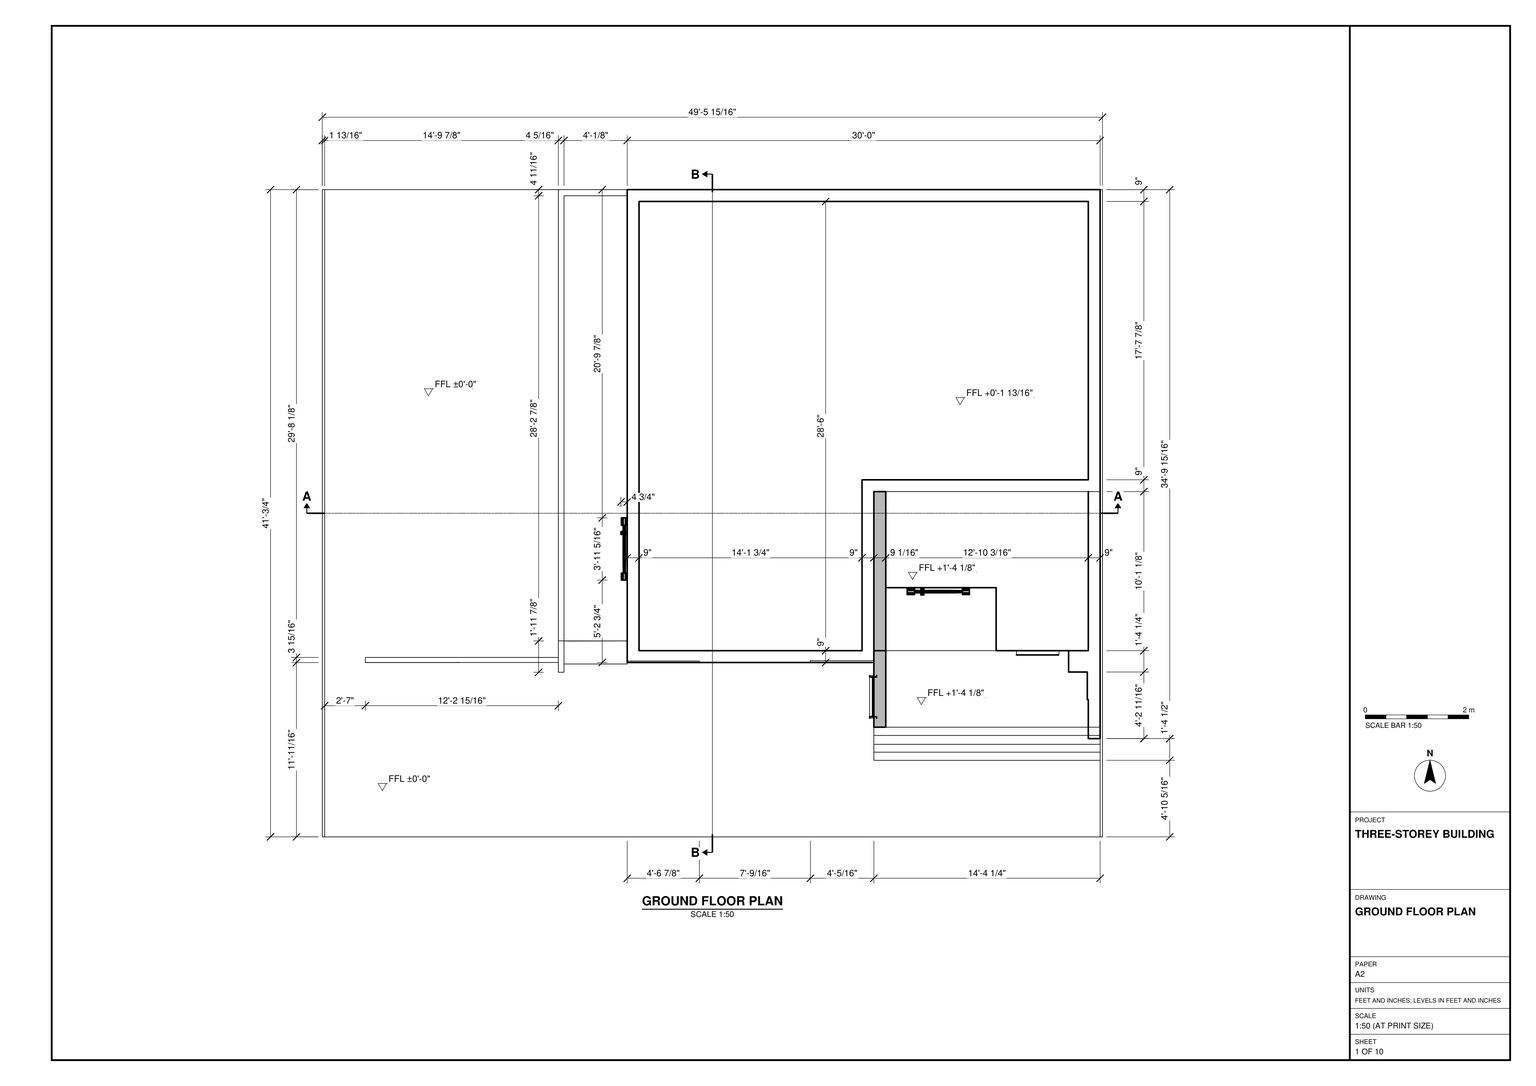
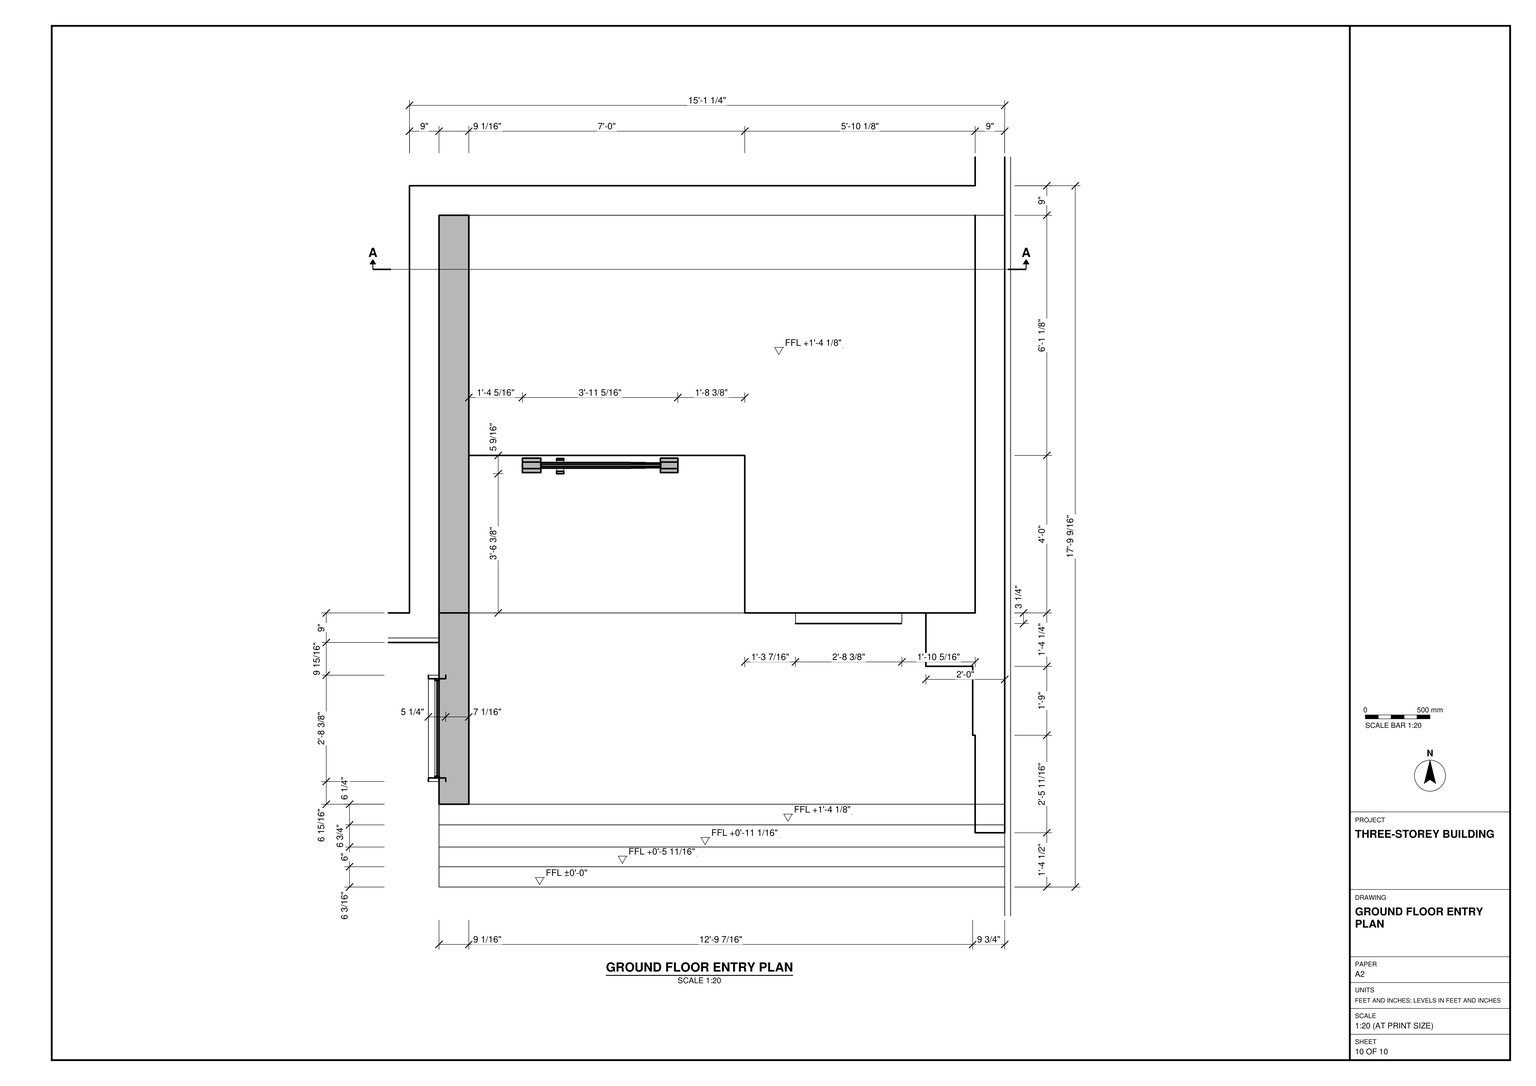
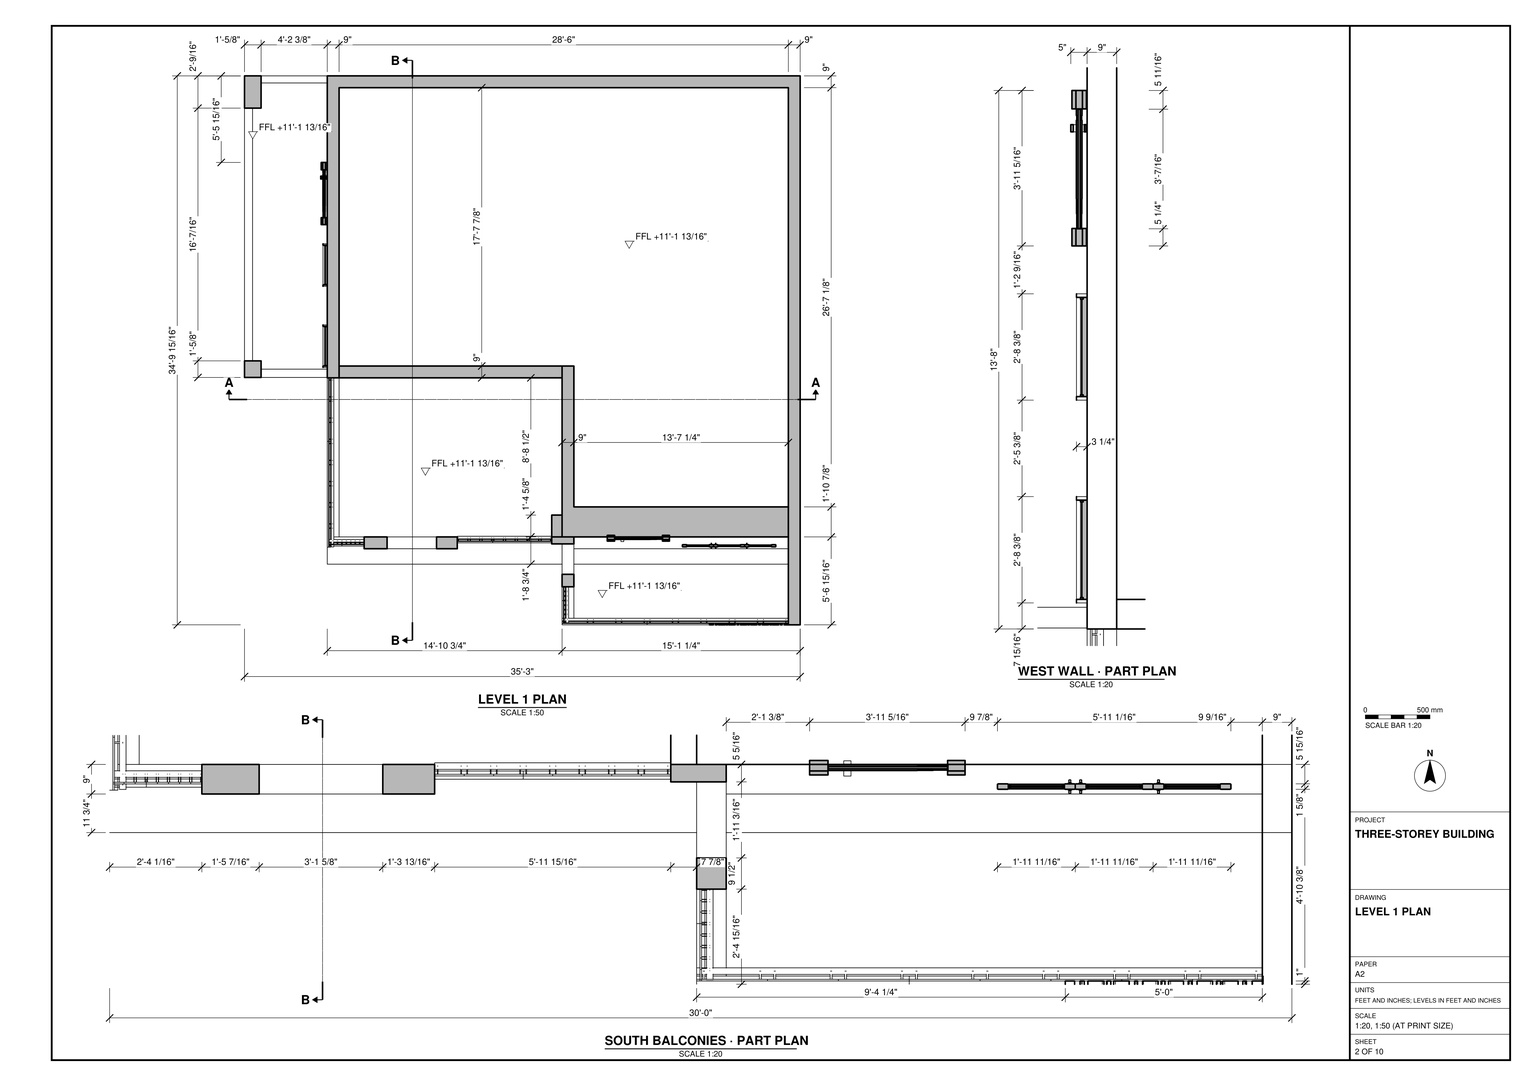
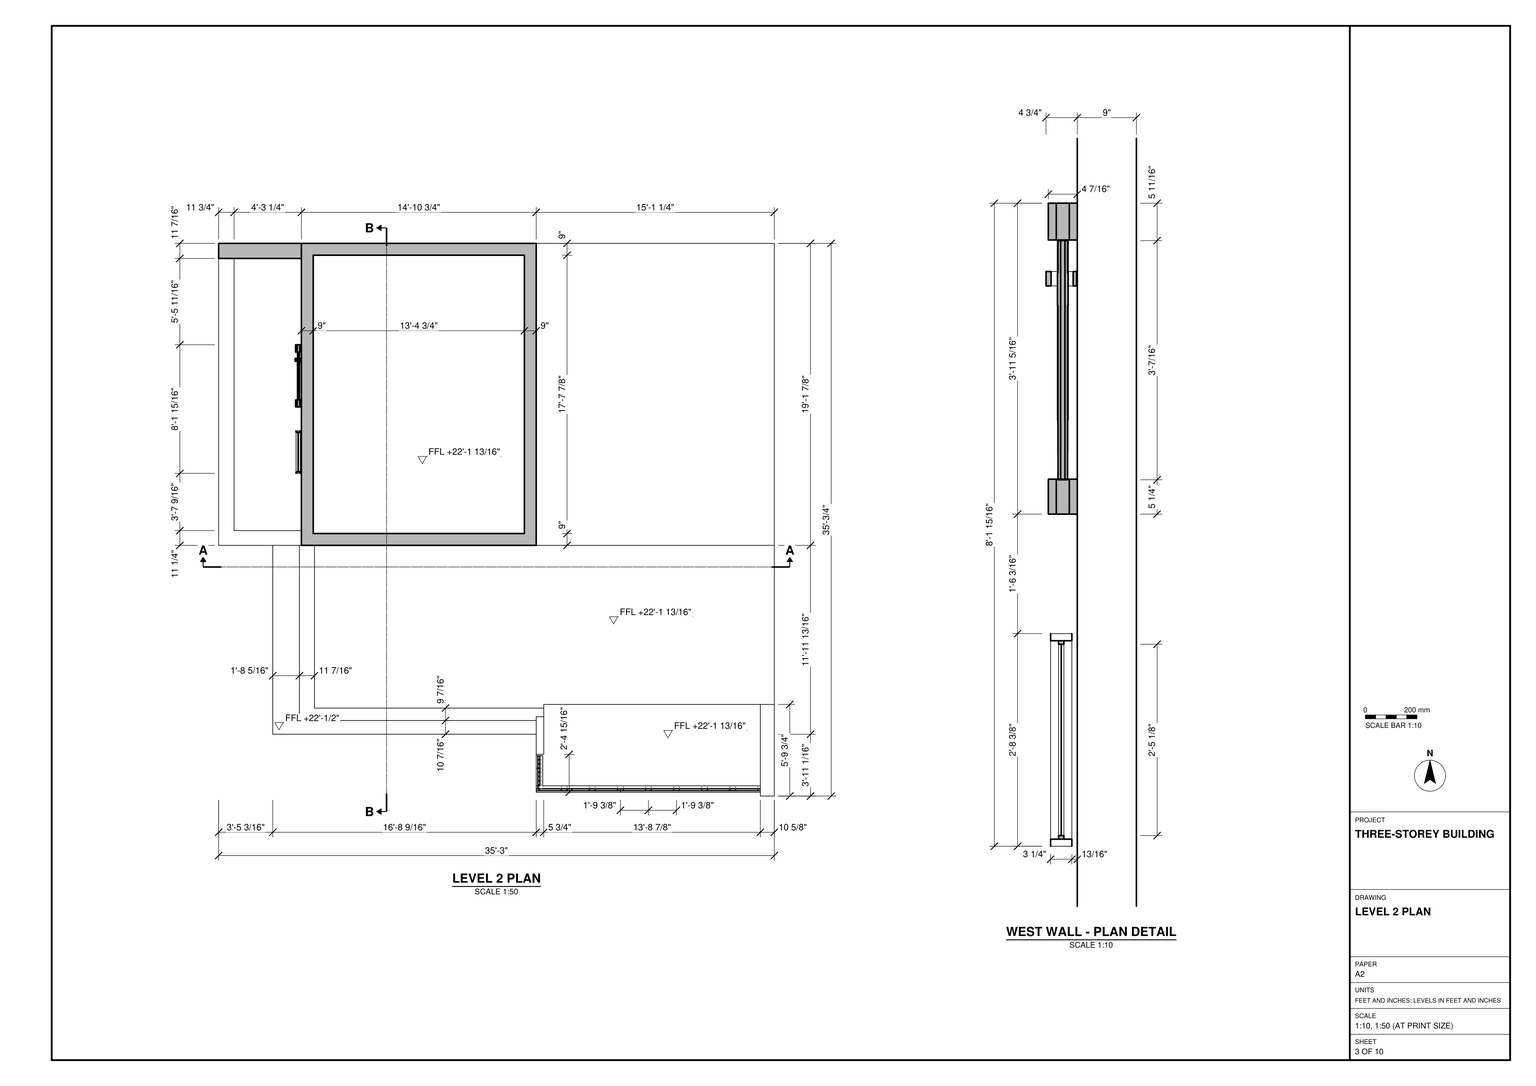
Build the three-storey building and its surrounding ground in SketchUp using task_files/diagram_01.pdf. Work in feet and inches. The overall model, including the ground shown in plan, measures 49'-5 15/16" along x, 41'-3/4" along y and 34'-0" along z. Use ±0'-0" as the ground datum and set the upper floor levels at +11'-1 13/16" and +22'-1 13/16".

Place the building on the east side of the ground plan, leaving the open area to the west. Use the enlarged entry plan to shape the south approach, steps and raised landing. Model the slabs and walls with their offsets, returns and thicknesses as drawn. On Level 1, follow the L-shaped enclosed area and the staggered outlines of the south balconies. Use the part plans to position the balcony guards, doors and window units. Follow the sheets for the uppermost storey, roof, stairs and any built-in joinery or main furniture shown. Suitable library components may be used for decor and loose items.

Keep shell elements such as walls, slabs and roof separate as groups or components. Do the same for each furniture or joinery piece, and use components for repeated parts. Save one SketchUp model as output_files/three_storey_building_with_south_balconies.skp.

# SketchUp Ruby script. Lengths in inches.
U = 1.inch
M = Sketchup.active_model
def pt(a) = Geom::Point3d.new(a.map { |v| v * U })
def face(e, loops, mat)
  f = e.add_face(loops[0].map { |a| pt(a) })
  loops[1..].each { |l| e.add_face(l.map { |a| pt(a) }).erase! }
  f.material = f.back_material = mat if mat
  f
end
# faces: each face lists its corners as indices into pts; further lists are holes
def faces(e, pts, list, mat = nil) = list.each { |f| face(e, (f[0].is_a?(Array) ? f : [f]).map { |l| l.map { |i| pts[i] } }, mat) }
# xy, xz, yz: faces in a plane at the given z, y or x. An outline is a flat list of corners, or four numbers for a rectangle; further outlines are holes
def ring(l) = l.size == 4 ? [[l[0], l[1]], [l[2], l[1]], [l[2], l[3]], [l[0], l[3]]] : l.each_slice(2).to_a
def flat(e, list, mat, &to3) = list.each { |f| face(e, (f[0].is_a?(Array) ? f : [f]).map { |l| ring(l).map { |u, v| to3.(u, v) } }, mat) }
def xy(e, z, list, mat = nil) = flat(e, list, mat) { |x, y| [x, y, z] }
def xz(e, y, list, mat = nil) = flat(e, list, mat) { |x, z| [x, y, z] }
def yz(e, x, list, mat = nil) = flat(e, list, mat) { |y, z| [x, y, z] }
def lines(e, pts, list) = list.each { |a, b| e.add_line(pt(pts[a]), pt(pts[b])) }
# prism: a flat outline (further loops are holes) pulled along v
def prism(e, loops, v, mat = nil)
  f = face(e, loops, mat); d = Geom::Vector3d.new(v.map { |x| x * U })
  f.pushpull(f.normal.samedirection?(d) ? d.length : -d.length)
end
def box(e, o, s, mat = nil) = prism(e, [[o, [o[0] + s[0], o[1], o[2]], [o[0] + s[0], o[1] + s[1], o[2]], [o[0], o[1] + s[1], o[2]]]], [0, 0, s[2]], mat)
def at(x, y, z, deg = 0) = Geom::Transformation.translation(pt([x, y, z])) * Geom::Transformation.rotation(ORIGIN, Z_AXIS, deg.degrees)
def axes(o, x, y, z) = Geom::Transformation.new([*x, 0, *y, 0, *z, 0, *pt(o).to_a, 1])
def part(name) = M.definitions.add(name)
# library, detail: a bought-in or finely detailed component or shape, given as its bounding box
def library(name, o, s) = part(name).tap { |d| box(d.entities, o, s) }
def detail(e, o, s) = box(e.add_group.entities, o, s)
def put(e, d, t, mat = nil) = e.add_instance(d, t).tap { |i| i.material = mat if mat }
def group(e, t, mat = nil) = e.add_group.tap { |g| g.transformation = t; g.material = mat if mat }.entities
root = M.entities
M.materials.add("[Color M00]1").color = [255, 255, 255]
M.materials.add("[Color M04]").color = [142, 142, 142]
M.materials.add("[Color M05]1").color = [114, 114, 114]
M.materials.add("[Color M06]").color = [86, 86, 86]
M.materials.add("[Color M08]1").color = [30, 30, 30]
M.materials.add("[Color M09]1").color = [0, 0, 0]
M.materials.add("[Wood Cherry Original]").color = [152, 86, 42]
M.materials.add("[Wood Floor Light]").color = [204, 176, 127]
M.materials.add("[Wood Veneer 01]").color = [120, 70, 37]
c1 = library("Three panel window",[0,0,0],[5.02,84.63,60])
c2 = library("PORTA PIVOTANTE D luxury",[0,-0.8125,0],[63.375,11.25,89])
c3 = library("Single panel window",[84,-6,0],[60,6,73.01])
c4 = library("Untitled",[0,0,0],[571,5,42])
c5 = library("jali pattern 5",[0,0,0],[60,1,120])
c6 = part("Group\#2")
xy(c6.entities,0,[[-232.125,-492.75,360,0]])
xy(c6.entities,10.1875,[[-232.125,-492.75,360,0]])
xz(c6.entities,-492.75,[[-232.125,0,360,10.1875]],"[Color M05]1")
xz(c6.entities,0,[[-232.125,0,360,10.1875]])
yz(c6.entities,-232.125,[[-492.75,0,0,10.1875]])
yz(c6.entities,360,[[-492.75,0,0,10.1875]])
c7 = part("Group\#7")
box(c7.entities,[0,0,0],[1.0625,3.0625,13.875])
xy(root,-12,[[419.875,58.28,592.125,83.5],[419.875,83.5,592.125,132.75]])
xy(root,-1.8125,[[419.875,58.28,592.125,64.47],[179.6875,125.3125,184,132.75],[32.78,132.6875,104.61,135.75],[105.04,132.75,179.6875,135.75],[184,488.08,232.125,492.75]])
xy(root,0,[[241.125,141.75,410.875,141.75,410.875,271.85,583.125,271.85,583.125,483.75,241.125,483.75]])
xy(root,3.875,[[419.875,64.47,592.125,70.47]])
xy(root,9.25,[[419.875,70.47,592.125,77.22]])
xy(root,14.3125,[[419.875,77.22,583.125,83.5],[428.95,83.5,583.125,83.5,583.125,104.5,582.375,104.5,582.375,125.5,568.125,125.5,568.125,141.75,428.95,141.75],[428.95,141.75,512.97,189.73],[512.97,141.75,583.125,141.75,583.125,262.85,428.95,262.85,428.95,189.73,512.97,189.73]])
xy(root,14.3125,[[583.125,74.8125,592.125,77.22]],"[Wood Floor Light]")
xy(root,18.25,[[32.78,132.6875,101.22,135.75],[102.28,132.6875,103.16,135.75],[105.04,132.75,106.54,135.75],[106.54,132.75,107.9,135.75],[107.9,132.75,108.64,135.75],
  [108.64,132.75,109.65,135.75],[109.65,132.75,110.39,135.75],[110.39,132.75,111.65,135.75],[111.65,132.75,112.39,135.75],[112.39,132.75,113.59,135.75],
  [113.59,132.75,114.33,135.75],[114.33,132.75,115.4,135.75],[115.4,132.75,116.14,135.75],[116.14,132.75,117.4,135.75],[117.4,132.75,118.14,135.75],
  [118.14,132.75,119.4,135.75],[119.4,132.75,120.14,135.75],[120.14,132.75,121.53,135.75],[121.53,132.75,122.27,135.75],[122.27,132.75,123.59,135.75],
  [123.59,132.75,124.33,135.75],[124.33,132.75,125.65,135.75],[125.65,132.75,126.39,135.75],[126.39,132.75,127.4,135.75],[127.4,132.75,128.14,135.75],
  [128.14,132.75,129.34,135.75],[129.34,132.75,130.08,135.75],[130.08,132.75,131.34,135.75],[131.34,132.75,132.08,135.75],[132.08,132.75,133.34,135.75],
  [133.34,132.75,134.08,135.75],[134.08,132.75,135.28,135.75],[135.28,132.75,136.02,135.75],[136.02,132.75,137.21,135.75],[137.21,132.75,137.95,135.75],
  [137.95,132.75,139.28,135.75],[139.28,132.75,140.02,135.75],[140.02,132.75,141.15,135.75],[141.15,132.75,141.89,135.75],[141.89,132.75,142.9,135.75],
  [142.9,132.75,143.64,135.75],[143.64,132.75,144.96,135.75],[144.96,132.75,145.7,135.75],[145.7,132.75,147.15,135.75],[147.15,132.75,147.89,135.75],
  [147.89,132.75,149.09,135.75],[149.09,132.75,149.83,135.75],[149.83,132.75,151.03,135.75],[151.03,132.75,151.77,135.75],[151.77,132.75,153.09,135.75],
  [153.09,132.75,153.83,135.75],[153.83,132.75,155.03,135.75],[155.03,132.75,155.77,135.75],[155.77,132.75,156.96,135.75],[156.96,132.75,157.7,135.75],
  [157.7,132.75,159.15,135.75],[159.15,132.75,159.89,135.75],[159.89,132.75,161.21,135.75],[161.21,132.75,161.95,135.75],[161.95,132.75,163.53,135.75],
  [163.53,132.75,164.27,135.75],[164.27,132.75,165.65,135.75],[165.65,132.75,166.39,135.75],[166.39,132.75,167.9,135.75],[167.9,132.75,168.64,135.75],
  [168.64,132.75,170.03,135.75],[170.03,132.75,170.77,135.75],[170.77,132.75,172.21,135.75],[172.21,132.75,172.95,135.75],[172.95,132.75,174.65,135.75],
  [174.65,132.75,175.39,135.75],[175.39,132.75,176.84,135.75],[176.84,132.75,177.58,135.75],[177.58,132.75,178.63,135.75],[178.63,132.75,179.375,135.75],
  [179.375,132.75,179.6875,135.75]])
xy(root,20.76,[[371.58,132.75,419.875,134.125]],"[Color M09]1")
xy(root,22.43,[[184,132.75,232.125,133.875],[232.125,132.75,287.02,133.875]],"[Color M09]1")
xy(root,23.37,[[371.58,132.75,419.875,134.125]],"[Color M09]1")
xy(root,24.34,[[184,132.75,232.125,133.875],[232.125,132.75,287.02,133.875]],"[Color M09]1")
xy(root,32.16,[[32.78,132.6875,103.16,135.75]])
xy(root,32.95,[[106.54,132.75,107.9,135.75],[107.9,132.75,108.64,135.75],[108.64,132.75,109.65,135.75],[109.65,132.75,110.39,135.75],[110.39,132.75,111.65,135.75],
  [111.65,132.75,112.39,135.75],[112.39,132.75,113.59,135.75],[113.59,132.75,114.33,135.75],[114.33,132.75,115.4,135.75],[115.4,132.75,116.14,135.75],
  [116.14,132.75,117.4,135.75],[117.4,132.75,118.14,135.75],[118.14,132.75,119.4,135.75],[119.4,132.75,120.14,135.75],[120.14,132.75,121.53,135.75],
  [121.53,132.75,122.27,135.75],[122.27,132.75,123.59,135.75],[123.59,132.75,124.33,135.75],[124.33,132.75,125.65,135.75],[125.65,132.75,126.39,135.75],
  [126.39,132.75,127.4,135.75],[127.4,132.75,128.14,135.75],[128.14,132.75,129.34,135.75],[129.34,132.75,130.08,135.75],[130.08,132.75,131.34,135.75],
  [131.34,132.75,132.08,135.75],[132.08,132.75,133.34,135.75],[133.34,132.75,134.08,135.75],[134.08,132.75,135.28,135.75],[135.28,132.75,136.02,135.75],
  [136.02,132.75,137.21,135.75],[137.21,132.75,137.95,135.75],[137.95,132.75,139.28,135.75],[139.28,132.75,140.02,135.75],[140.02,132.75,141.15,135.75],
  [141.15,132.75,141.89,135.75],[141.89,132.75,142.9,135.75],[142.9,132.75,143.64,135.75],[143.64,132.75,144.96,135.75],[144.96,132.75,145.7,135.75],
  [145.7,132.75,147.15,135.75],[147.15,132.75,147.89,135.75],[147.89,132.75,149.09,135.75],[149.09,132.75,149.83,135.75],[149.83,132.75,151.03,135.75],
  [151.03,132.75,151.77,135.75],[151.77,132.75,153.09,135.75],[153.09,132.75,153.83,135.75],[153.83,132.75,155.03,135.75],[155.03,132.75,155.77,135.75],
  [155.77,132.75,156.96,135.75],[156.96,132.75,157.7,135.75],[157.7,132.75,159.15,135.75],[159.15,132.75,159.89,135.75],[159.89,132.75,161.21,135.75],
  [161.21,132.75,161.95,135.75],[161.95,132.75,163.53,135.75],[163.53,132.75,164.27,135.75],[164.27,132.75,165.65,135.75],[165.65,132.75,166.39,135.75],
  [166.39,132.75,167.9,135.75],[167.9,132.75,168.64,135.75],[168.64,132.75,170.03,135.75],[170.03,132.75,170.77,135.75],[170.77,132.75,172.21,135.75],
  [172.21,132.75,172.95,135.75],[172.95,132.75,174.65,135.75],[174.65,132.75,175.39,135.75],[175.39,132.75,176.84,135.75],[176.84,132.75,177.58,135.75],
  [177.58,132.75,178.63,135.75],[178.63,132.75,179.375,135.75],[179.375,132.75,179.6875,135.75]])
xy(root,34.1875,[[103.16,132.75,105.04,135.75],[32.78,135.75,179.6875,136.625]])
xy(root,34.1875,[[32.78,132.6875,103.16,132.75],[32.78,132.75,103.16,135.75],[105.04,132.75,179.6875,135.75]],"[Color M08]1")
xy(root,38.9375,[[32.78,132.75,179.6875,136.625]])
xy(root,44.125,[[184,131.625,232.125,132.75],[184,132.75,232.125,149.1875]])
xy(root,45.375,[[179.6875,125.3125,184,149.1875],[184,131.625,232.125,149.1875],[179.6875,149.1875,184,149.1875,184,488.08,232.125,488.08,232.125,492.75,179.6875,492.75]])
xy(root,120,[[410.875,74.8125,419.875,132.75],[419.875,74.8125,419.875,83.5,428.95,83.5,428.95,132.75,568.125,132.75,568.125,125.5,583.125,125.5,583.125,74.8125],[583.125,74.8125,592.125,132.75],[419.875,83.5,428.95,132.75],[568.125,125.5,583.125,132.75],
  [[232.125,132.75,419.875,132.75,419.875,262.85,428.95,262.85,428.95,189.73,512.97,189.73,512.97,141.75,583.125,141.75,583.125,262.85,592.125,262.85,592.125,492.75,232.125,492.75],[241.125,141.75,241.125,483.75,583.125,483.75,583.125,271.85,410.875,271.85,410.875,141.75]],[419.875,132.75,428.95,141.75],[568.125,132.75,583.125,141.75],[583.125,132.75,592.125,262.85],[419.875,141.75,428.95,262.85],
  [169.125,263.15,232.125,492.75]])
xy(root,132,[[410.875,74.8125,419.875,103.78],[419.875,74.8125,583.125,132.75],[260.21,132.75,277.66,141.75],[277.66,132.75,315.3,141.75],[315.3,132.75,331.09,141.75],
  [419.875,132.75,583.125,141.75],[403,136.4375,410.875,141.75],[232.125,141.75,241.125,262.85],[241.125,141.75,403,141.75,403,158.375,410.875,158.375,410.875,262.85,241.125,262.85],[410.875,141.75,583.125,141.75,583.125,164.6,419.875,164.6,419.875,271.85,410.875,271.85],
  [583.125,141.75,592.125,262.85],[419.875,164.6,583.125,164.6,583.125,483.75,241.125,483.75,241.125,271.85,419.875,271.85],[232.125,262.85,241.125,262.85,241.125,483.75,583.125,483.75,583.125,262.85,592.125,262.85,592.125,492.75,232.125,492.75],[181.75,269.46,232.125,269.46,232.125,487.34,181.75,487.34,181.75,468.1875,175.25,468.1875,175.25,275.78,181.75,275.78]])
xy(root,151.1875,[[277.66,132.75,315.3,141.75]])
xy(root,158.375,[[181.75,263.15,232.125,269.46],[169.125,275.78,175.25,468.1875],[181.75,487.34,232.125,492.75]])
xy(root,171.5625,[[410.875,113.28,419.875,136.4375]])
xy(root,237.625,[[169.125,275.78,181.75,468.1875]])
xy(root,241.7,[[410.875,113.28,419.875,136.4375]])
xy(root,251.51,[[403,141.75,410.875,158.375]])
xy(root,252,[[410.875,74.8125,419.875,103.78],[419.875,74.8125,583.125,141.75],[212.25,120.6875,212.25,132.4375,331.09,132.4375,331.09,141.75,315.3,141.75,315.3,132.4375,277.66,132.4375,277.66,141.75,260.21,141.75,260.21,132.4375,232.125,132.4375,232.125,262.85,410.875,262.85,410.875,141.75,403,141.75,403,136.4375,410.875,136.4375,410.875,120.6875],[583.125,132.75,592.125,141.75],[410.875,141.75,419.875,262.85],
  [419.875,141.75,583.125,164.6],[583.125,141.75,592.125,262.85],[419.875,164.6,583.125,262.85],[169.125,262.85,169.125,263.15,181.75,263.15,181.75,492.75,232.125,492.75,232.125,262.85],[232.125,262.85,241.125,262.85,241.125,483.75,583.125,483.75,583.125,262.85,592.125,262.85,592.125,492.75,232.125,492.75],
  [241.125,262.85,410.875,271.85],[419.875,262.85,583.125,262.85,583.125,483.75,241.125,483.75,241.125,271.85,419.875,271.85],[410.875,262.85,419.875,271.85]])
xy(root,252.25,[[212.25,132.4375,232.125,266.25],[260.21,132.4375,277.66,132.75],[315.3,132.4375,331.09,132.75],[260.21,132.75,277.66,141.75],[315.3,132.75,331.09,141.75]])
xy(root,260.88,[[210.3125,119.0625,212.25,262.85],[212.25,119.0625,410.875,120.6875]])
xy(root,262.6875,[[210.3125,119.0625,410.875,119.0625,410.875,132.4375,232.125,132.4375,232.125,266.25,212.25,266.25,212.25,262.85,210.3125,262.85]])
xy(root,264,[[410.875,74.8125,583.125,74.8125,583.125,141.75,416.625,141.75,416.625,103.78,410.875,103.78],[242.08,138.97,416.625,138.97,416.625,141.75,592.125,141.75,592.125,262.85,242.08,262.85],[169.125,262.85,232.125,262.85,232.125,274.08,180.875,274.08,180.875,481.29,232.125,481.29,232.125,492.75,169.125,492.75],[241.125,271.85,401.875,483.75],[180.875,274.08,232.125,481.29]])
xy(root,295.15,[[169.125,262.85,232.125,262.85,232.125,274.08,180.875,274.08,180.875,481.29,169.125,481.29]])
xy(root,298.5625,[[581.5,72,592.125,74.8125],[581.5,74.8125,583.125,141.75],[583.125,74.8125,592.125,141.75]],"[Wood Floor Light]")
xy(root,298.875,[[410.875,103.78,416.625,132.4375],[230.625,129.5,232.125,262.85],[232.125,129.5,410.875,132.4375],[232.125,132.4375,232.125,262.85,242.08,262.85,242.08,138.97,416.625,138.97,416.625,132.4375]])
xy(root,300.5625,[[581.5,72,592.125,141.75]],"[Wood Floor Light]")
xy(root,300.625,[[230.625,129.5,410.875,129.5,410.875,132.4375,416.625,132.4375,416.625,138.97,242.08,138.97,242.08,262.85,230.625,262.85]])
xy(root,334.45,[[325.42,252.1,400.04,262.85]],"[Color M00]1")
xy(root,340.7,[[325.42,252.1,400.04,262.85]],"[Color M00]1")
xy(root,373.9375,[[169.125,262.85,232.125,481.29]])
xy(root,384,[[[232.125,262.85,410.875,492.75],[241.125,271.85,401.875,483.75]]])
xy(root,396,[[169.125,262.85,232.125,262.85,232.125,492.75,208.8125,492.75,208.8125,481.29,169.125,481.29],[169.125,481.29,208.8125,492.75]])
xz(root,58.28,[[419.875,-12,592.125,-1.8125]],"[Color M04]")
xz(root,64.47,[[419.875,-1.8125,592.125,3.875]],"[Color M04]")
xz(root,70.47,[[419.875,3.875,592.125,9.25]],"[Color M04]")
xz(root,72,[[581.5,298.5625,592.125,300.5625]],"[Wood Floor Light]")
xz(root,74.8125,[[410.875,120,419.875,132],[419.875,120,583.125,132],[410.875,252,583.125,264]])
xz(root,74.8125,[[583.125,14.3125,592.125,120],[583.125,120,592.125,298.5625]],"[Wood Floor Light]")
xz(root,77.22,[[419.875,9.25,592.125,14.3125]],"[Color M04]")
xz(root,83.5,[[419.875,14.3125,428.95,120]])
xz(root,103.78,[[410.875,132,419.875,252],[410.875,264,416.625,298.875]])
xz(root,104.5,[[582.375,14.3125,583.125,52.76]])
xz(root,113.28,[[410.875,171.5625,419.875,241.7]])
xz(root,119.0625,[[210.3125,260.88,410.875,262.6875]])
xz(root,120.6875,[[212.25,252,410.875,260.88]])
xz(root,125.3125,[[179.6875,-1.8125,184,45.375]])
xz(root,125.5,[[568.125,14.3125,582.375,14.3125,582.375,54.32,583.125,54.32,583.125,120,568.125,120]],"[Wood Floor Light]")
xz(root,129.5,[[230.625,298.875,410.875,300.625]])
xz(root,131.625,[[184,44.125,232.125,45.375]])
xz(root,132.4375,[[212.25,252,232.125,252.25],[232.125,252,260.21,252.25],[260.21,252,277.66,252.25],[277.66,252,315.3,252.25],[315.3,252,331.09,252.25],
  [232.125,262.6875,410.875,298.875],[410.875,298.875,416.625,300.625]])
xz(root,132.6875,[[32.78,-1.8125,104.61,18.25]],"[Color M05]1")
xz(root,132.6875,[[32.78,32.16,103.16,34.1875]],"[Color M08]1")
xz(root,132.75,[[184,-1.8125,232.125,22.43],[287.02,-1.8125,371.58,32.48],[184,24.34,232.125,44.125],[32.78,34.1875,179.6875,38.9375],[287.02,61.92,371.58,120],
  [277.66,132,315.3,151.1875]])
xz(root,132.75,[[105.04,-1.8125,179.6875,18.25],[232.125,-1.8125,287.02,22.43],[371.58,-1.8125,419.875,20.76],[371.58,23.37,419.875,120],[232.125,24.34,287.02,120]],"[Color M05]1")
xz(root,132.75,[[260.21,132,277.66,252.25],[315.3,132,331.09,252.25]],"[Color M06]")
xz(root,132.75,[[105.04,18.25,106.54,18.25,106.54,32.95,179.6875,32.95,179.6875,34.1875,105.04,34.1875],[107.9,18.25,108.64,32.95],[109.65,18.25,110.39,32.95],[111.65,18.25,112.39,32.95],[113.59,18.25,114.33,32.95],
  [115.4,18.25,116.14,32.95],[117.4,18.25,118.14,32.95],[119.4,18.25,120.14,32.95],[121.53,18.25,122.27,32.95],[123.59,18.25,124.33,32.95],
  [125.65,18.25,126.39,32.95],[127.4,18.25,128.14,32.95],[129.34,18.25,130.08,32.95],[131.34,18.25,132.08,32.95],[133.34,18.25,134.08,32.95],
  [135.28,18.25,136.02,32.95],[137.21,18.25,137.95,32.95],[139.28,18.25,140.02,32.95],[141.15,18.25,141.89,32.95],[142.9,18.25,143.64,32.95],
  [144.96,18.25,145.7,32.95],[147.15,18.25,147.89,32.95],[149.09,18.25,149.83,32.95],[151.03,18.25,151.77,32.95],[153.09,18.25,153.83,32.95],
  [155.03,18.25,155.77,32.95],[156.96,18.25,157.7,32.95],[159.15,18.25,159.89,32.95],[161.21,18.25,161.95,32.95],[163.53,18.25,164.27,32.95],
  [165.65,18.25,166.39,32.95],[167.9,18.25,168.64,32.95],[170.03,18.25,170.77,32.95],[172.21,18.25,172.95,32.95],[174.65,18.25,175.39,32.95],
  [176.84,18.25,177.58,32.95],[178.63,18.25,179.375,32.95],[[287.02,32.48,371.58,61.92],[351.3,33.48,370.58,60.92],[309.11,33.48,328.21,60.92],[288.02,33.48,307.11,60.92],[330.21,33.48,349.3,60.92]]],"[Color M08]1")
xz(root,132.75,[[288.02,33.48,307.11,60.92],[309.11,33.48,328.21,60.92],[330.21,33.48,349.3,60.92],[351.3,33.48,370.58,60.92]],"[Wood Cherry Original]")
xz(root,133.875,[[184,22.43,232.125,24.34],[232.125,22.43,287.02,24.34]],"[Color M09]1")
xz(root,134.125,[[371.58,20.76,419.875,23.37]],"[Color M09]1")
xz(root,135.75,[[32.78,-1.8125,104.61,18.25],[105.04,-1.8125,179.6875,18.25]],"[Color M05]1")
xz(root,135.75,[[105.04,18.25,105.04,34.1875,179.6875,34.1875,179.6875,32.95,106.54,32.95,106.54,18.25],[107.9,18.25,108.64,32.95],[109.65,18.25,110.39,32.95],[111.65,18.25,112.39,32.95],[113.59,18.25,114.33,32.95],
  [115.4,18.25,116.14,32.95],[117.4,18.25,118.14,32.95],[119.4,18.25,120.14,32.95],[121.53,18.25,122.27,32.95],[123.59,18.25,124.33,32.95],
  [125.65,18.25,126.39,32.95],[127.4,18.25,128.14,32.95],[129.34,18.25,130.08,32.95],[131.34,18.25,132.08,32.95],[133.34,18.25,134.08,32.95],
  [135.28,18.25,136.02,32.95],[137.21,18.25,137.95,32.95],[139.28,18.25,140.02,32.95],[141.15,18.25,141.89,32.95],[142.9,18.25,143.64,32.95],
  [144.96,18.25,145.7,32.95],[147.15,18.25,147.89,32.95],[149.09,18.25,149.83,32.95],[151.03,18.25,151.77,32.95],[153.09,18.25,153.83,32.95],
  [155.03,18.25,155.77,32.95],[156.96,18.25,157.7,32.95],[159.15,18.25,159.89,32.95],[161.21,18.25,161.95,32.95],[163.53,18.25,164.27,32.95],
  [165.65,18.25,166.39,32.95],[167.9,18.25,168.64,32.95],[170.03,18.25,170.77,32.95],[172.21,18.25,172.95,32.95],[174.65,18.25,175.39,32.95],
  [176.84,18.25,177.58,32.95],[178.63,18.25,179.375,32.95],[32.78,32.16,103.16,34.1875]],"[Color M08]1")
xz(root,136.4375,[[403,132,410.875,132,410.875,171.5625,419.875,171.5625,419.875,241.7,410.875,241.7,410.875,252,403,252]],"[Wood Veneer 01]")
xz(root,136.625,[[32.78,34.1875,179.6875,38.9375]])
xz(root,138.97,[[242.08,264,410.875,298.875],[410.875,264,416.625,298.875],[242.08,298.875,410.875,300.625],[410.875,298.875,416.625,300.625]])
xz(root,141.75,[[241.125,0,410.875,120],[419.875,0,419.875,120,428.95,120,428.95,14.3125,583.125,14.3125,583.125,0],[512.97,14.3125,568.125,120],[568.125,14.3125,583.125,120],[260.21,132,277.66,252],
  [277.66,132,315.3,151.1875],[315.3,132,331.09,252],[403,132,410.875,251.51],[410.875,132,419.875,171.5625],[410.875,171.5625,419.875,220.01],
  [410.875,220.01,419.875,252],[403,251.51,410.875,252],[260.21,252,277.66,252.25],[315.3,252,331.09,252.25],[583.125,264,592.125,271.1875],
  [583.125,271.1875,592.125,298.5625]])
xz(root,141.75,[[419.875,132,583.125,252],[581.5,298.5625,592.125,300.5625]],"[Wood Floor Light]")
xz(root,149.1875,[[180.35,-1.8125,184,45.375],[184,0,232.125,44.125],[184,44.125,232.125,45.375]])
xz(root,158.375,[[403,132,410.875,251.51]])
xz(root,164.6,[[419.875,132,583.125,252]])
xz(root,189.73,[[428.95,14.3125,512.97,120]])
xz(root,252.1,[[325.42,334.45,400.04,340.7]],"[Color M00]1")
xz(root,262.85,[[419.875,0,583.125,0,583.125,14.3125,428.95,14.3125,428.95,120,419.875,120],[232.125,132,241.125,252],[232.125,252,232.125,298.875,242.08,298.875,242.08,264,592.125,264,592.125,252],[210.3125,260.88,212.25,262.6875],[169.125,264,232.125,295.15],
  [230.625,298.875,232.125,300.625],[232.125,298.875,242.08,300.625],[169.125,373.9375,232.125,396]])
xz(root,262.85,[[169.125,252,232.125,264],[242.08,264,260.87,264,260.87,384,232.125,384,232.125,300.625,242.08,300.625],[[304.55,264,410.875,384],[325.42,334.45,400.04,340.7]]],"[Color M06]")
xz(root,262.85,[[241.125,132,410.875,252],[260.87,264,304.55,384],[260.87,384,304.55,396]],"[Wood Floor Light]")
xz(root,263.15,[[181.75,132,232.125,158.375]])
xz(root,263.15,[[169.125,120,232.125,120,232.125,132,181.75,132,181.75,252,169.125,252]],"[Color M06]")
xz(root,266.25,[[212.25,252.25,232.125,262.6875]])
xz(root,269.46,[[181.75,132,232.125,158.375]])
xz(root,271.85,[[410.875,0,583.125,120],[241.125,132,410.875,252],[410.875,132,419.875,252],[241.125,264,401.875,384]])
xz(root,274.08,[[180.875,264,232.125,295.15]])
xz(root,275.78,[[175.25,132,175.25,158.375,169.125,158.375,169.125,237.625,181.75,237.625,181.75,132]])
xz(root,468.1875,[[175.25,132,181.75,152.3125],[175.25,152.3125,181.75,152.3125,181.75,237.625,169.125,237.625,169.125,158.375,175.25,158.375]])
xz(root,481.29,[[180.875,264,232.125,264,232.125,373.9375,169.125,373.9375,169.125,295.15,180.875,295.15]])
xz(root,483.75,[[241.125,0,583.125,120],[241.125,132,583.125,252],[241.125,264,401.875,384]])
xz(root,487.34,[[181.75,132,232.125,158.375]])
xz(root,488.08,[[184,-1.8125,232.125,45.375]])
xz(root,492.75,[[179.6875,-1.8125,232.125,45.375],[232.125,-1.8125,592.125,120],[232.125,132,592.125,252],[169.125,264,232.125,396],[232.125,264,410.875,384]])
xz(root,492.75,[[169.125,120,232.125,132],[169.125,132,169.125,264,232.125,264,232.125,252,181.75,252,181.75,158.375,193.6875,158.375,193.6875,132],[193.6875,132,232.125,158.375]],"[Color M06]")
yz(root,32.78,[[132.75,34.1875,136.625,38.9375]])
yz(root,32.78,[[132.6875,-1.8125,135.75,18.25]],"[Color M05]1")
yz(root,32.78,[[132.6875,32.16,135.75,34.1875]],"[Color M08]1")
yz(root,103.16,[[132.6875,32.16,135.75,34.1875]])
yz(root,104.61,[[132.6875,-1.8125,135.75,18.25]])
yz(root,105.04,[[132.75,-1.8125,135.75,18.25]],"[Color M05]1")
yz(root,105.04,[[132.75,18.25,135.75,34.1875]],"[Color M08]1")
yz(root,106.54,[[132.75,18.25,135.75,32.95]],"[Color M08]1")
yz(root,107.9,[[132.75,18.25,135.75,32.95]],"[Color M08]1")
yz(root,108.64,[[132.75,18.25,135.75,32.95]],"[Color M08]1")
yz(root,109.65,[[132.75,18.25,135.75,32.95]],"[Color M08]1")
yz(root,110.39,[[132.75,18.25,135.75,32.95]],"[Color M08]1")
yz(root,111.65,[[132.75,18.25,135.75,32.95]],"[Color M08]1")
yz(root,112.39,[[132.75,18.25,135.75,32.95]],"[Color M08]1")
yz(root,113.59,[[132.75,18.25,135.75,32.95]],"[Color M08]1")
yz(root,114.33,[[132.75,18.25,135.75,32.95]],"[Color M08]1")
yz(root,115.4,[[132.75,18.25,135.75,32.95]],"[Color M08]1")
yz(root,116.14,[[132.75,18.25,135.75,32.95]],"[Color M08]1")
yz(root,117.4,[[132.75,18.25,135.75,32.95]],"[Color M08]1")
yz(root,118.14,[[132.75,18.25,135.75,32.95]],"[Color M08]1")
yz(root,119.4,[[132.75,18.25,135.75,32.95]],"[Color M08]1")
yz(root,120.14,[[132.75,18.25,135.75,32.95]],"[Color M08]1")
yz(root,121.53,[[132.75,18.25,135.75,32.95]],"[Color M08]1")
yz(root,122.27,[[132.75,18.25,135.75,32.95]],"[Color M08]1")
yz(root,123.59,[[132.75,18.25,135.75,32.95]],"[Color M08]1")
yz(root,124.33,[[132.75,18.25,135.75,32.95]],"[Color M08]1")
yz(root,125.65,[[132.75,18.25,135.75,32.95]],"[Color M08]1")
yz(root,126.39,[[132.75,18.25,135.75,32.95]],"[Color M08]1")
yz(root,127.4,[[132.75,18.25,135.75,32.95]],"[Color M08]1")
yz(root,128.14,[[132.75,18.25,135.75,32.95]],"[Color M08]1")
yz(root,129.34,[[132.75,18.25,135.75,32.95]],"[Color M08]1")
yz(root,130.08,[[132.75,18.25,135.75,32.95]],"[Color M08]1")
yz(root,131.34,[[132.75,18.25,135.75,32.95]],"[Color M08]1")
yz(root,132.08,[[132.75,18.25,135.75,32.95]],"[Color M08]1")
yz(root,133.34,[[132.75,18.25,135.75,32.95]],"[Color M08]1")
yz(root,134.08,[[132.75,18.25,135.75,32.95]],"[Color M08]1")
yz(root,135.28,[[132.75,18.25,135.75,32.95]],"[Color M08]1")
yz(root,136.02,[[132.75,18.25,135.75,32.95]],"[Color M08]1")
yz(root,137.21,[[132.75,18.25,135.75,32.95]],"[Color M08]1")
yz(root,137.95,[[132.75,18.25,135.75,32.95]],"[Color M08]1")
yz(root,139.28,[[132.75,18.25,135.75,32.95]],"[Color M08]1")
yz(root,140.02,[[132.75,18.25,135.75,32.95]],"[Color M08]1")
yz(root,141.15,[[132.75,18.25,135.75,32.95]],"[Color M08]1")
yz(root,141.89,[[132.75,18.25,135.75,32.95]],"[Color M08]1")
yz(root,142.9,[[132.75,18.25,135.75,32.95]],"[Color M08]1")
yz(root,143.64,[[132.75,18.25,135.75,32.95]],"[Color M08]1")
yz(root,144.96,[[132.75,18.25,135.75,32.95]],"[Color M08]1")
yz(root,145.7,[[132.75,18.25,135.75,32.95]],"[Color M08]1")
yz(root,147.15,[[132.75,18.25,135.75,32.95]],"[Color M08]1")
yz(root,147.89,[[132.75,18.25,135.75,32.95]],"[Color M08]1")
yz(root,149.09,[[132.75,18.25,135.75,32.95]],"[Color M08]1")
yz(root,149.83,[[132.75,18.25,135.75,32.95]],"[Color M08]1")
yz(root,151.03,[[132.75,18.25,135.75,32.95]],"[Color M08]1")
yz(root,151.77,[[132.75,18.25,135.75,32.95]],"[Color M08]1")
yz(root,153.09,[[132.75,18.25,135.75,32.95]],"[Color M08]1")
yz(root,153.83,[[132.75,18.25,135.75,32.95]],"[Color M08]1")
yz(root,155.03,[[132.75,18.25,135.75,32.95]],"[Color M08]1")
yz(root,155.77,[[132.75,18.25,135.75,32.95]],"[Color M08]1")
yz(root,156.96,[[132.75,18.25,135.75,32.95]],"[Color M08]1")
yz(root,157.7,[[132.75,18.25,135.75,32.95]],"[Color M08]1")
yz(root,159.15,[[132.75,18.25,135.75,32.95]],"[Color M08]1")
yz(root,159.89,[[132.75,18.25,135.75,32.95]],"[Color M08]1")
yz(root,161.21,[[132.75,18.25,135.75,32.95]],"[Color M08]1")
yz(root,161.95,[[132.75,18.25,135.75,32.95]],"[Color M08]1")
yz(root,163.53,[[132.75,18.25,135.75,32.95]],"[Color M08]1")
yz(root,164.27,[[132.75,18.25,135.75,32.95]],"[Color M08]1")
yz(root,165.65,[[132.75,18.25,135.75,32.95]],"[Color M08]1")
yz(root,166.39,[[132.75,18.25,135.75,32.95]],"[Color M08]1")
yz(root,167.9,[[132.75,18.25,135.75,32.95]],"[Color M08]1")
yz(root,168.64,[[132.75,18.25,135.75,32.95]],"[Color M08]1")
yz(root,169.125,[[275.78,132,468.1875,158.375],[262.85,264,262.85,295.15,481.29,295.15,481.29,396,492.75,396,492.75,264],[262.85,373.9375,481.29,396]])
yz(root,169.125,[[263.15,120,263.15,252,275.78,252,275.78,132,492.75,132,492.75,120],[468.1875,132,468.1875,237.625,275.78,237.625,275.78,252,262.85,252,262.85,264,492.75,264,492.75,132]],"[Color M06]")
yz(root,170.03,[[132.75,18.25,135.75,32.95]],"[Color M08]1")
yz(root,170.77,[[132.75,18.25,135.75,32.95]],"[Color M08]1")
yz(root,172.21,[[132.75,18.25,135.75,32.95]],"[Color M08]1")
yz(root,172.95,[[132.75,18.25,135.75,32.95]],"[Color M08]1")
yz(root,174.65,[[132.75,18.25,135.75,32.95]],"[Color M08]1")
yz(root,175.25,[[275.78,132,468.1875,158.375]])
yz(root,175.39,[[132.75,18.25,135.75,32.95]],"[Color M08]1")
yz(root,176.84,[[132.75,18.25,135.75,32.95]],"[Color M08]1")
yz(root,177.58,[[132.75,18.25,135.75,32.95]],"[Color M08]1")
yz(root,178.63,[[132.75,18.25,135.75,32.95]],"[Color M08]1")
yz(root,179.375,[[132.75,18.25,135.75,32.95]],"[Color M08]1")
yz(root,179.6875,[[125.3125,-1.8125,132.75,0],[[135.75,-1.8125,135.75,18.25,132.75,18.25,132.75,0,125.3125,0,125.3125,45.375,492.75,45.375,492.75,-1.8125],[132.75,32.95,135.75,32.95,135.75,34.1875,136.625,34.1875,136.625,38.9375,132.75,38.9375]],[132.75,-1.8125,135.75,0],[132.75,0,135.75,18.25],[132.75,32.95,135.75,34.1875],
  [132.75,34.1875,136.625,38.9375]])
yz(root,180.875,[[274.08,264,481.29,295.15]])
yz(root,181.75,[[269.46,132,275.78,158.375],[468.1875,132,487.34,132,487.34,158.375,492.75,158.375,492.75,252,468.1875,252],[263.15,158.375,275.78,252],[275.78,237.625,468.1875,252]])
yz(root,184,[[125.3125,-1.8125,132.75,-1.8125,132.75,22.43,133.875,22.43,133.875,24.34,132.75,24.34,132.75,44.125,131.625,44.125,131.625,45.375,125.3125,45.375],[149.1875,-1.8125,488.08,45.375],[131.625,44.125,132.75,45.375],[132.75,44.125,149.1875,45.375]])
yz(root,210.3125,[[119.0625,260.88,262.85,262.6875]])
yz(root,212.25,[[120.6875,252,120.6875,260.88,262.85,260.88,262.85,262.6875,266.25,262.6875,266.25,252.25,132.4375,252.25,132.4375,252]])
yz(root,230.625,[[129.5,298.875,262.85,300.625]])
yz(root,232.125,[[488.08,-1.8125,492.75,0],[132.75,0,132.75,22.43,133.875,22.43,133.875,24.34,132.75,24.34,132.75,44.125,149.1875,44.125,149.1875,0],[149.1875,0,149.1875,45.375,132.75,45.375,132.75,120,492.75,120,492.75,45.375,488.08,45.375,488.08,0],[488.08,0,492.75,45.375],[131.625,44.125,132.75,45.375],
  [132.75,44.125,149.1875,45.375],[263.15,120,492.75,132],[262.85,132,262.85,252,492.75,252,492.75,158.375,487.34,158.375,487.34,132,269.46,132,269.46,158.375,263.15,158.375,263.15,132],[487.34,132,492.75,158.375],[132.4375,252,262.85,252.25],
  [262.85,252,492.75,252,492.75,264,262.85,264,262.85,262.6875,266.25,262.6875,266.25,252.25,262.85,252.25],[132.4375,252.25,262.85,262.6875],[262.85,252.25,266.25,262.6875],[132.4375,262.6875,262.85,298.875],[274.08,264,274.08,295.15,262.85,295.15,262.85,373.9375,481.29,373.9375,481.29,264],
  [481.29,264,481.29,373.9375,262.85,373.9375,262.85,384,492.75,384,492.75,264],[262.85,384,492.75,396]])
yz(root,241.125,[[141.75,0,483.75,120],[262.85,132,271.85,252],[271.85,132,483.75,252],[271.85,264,483.75,384]])
yz(root,242.08,[[138.97,264,262.85,298.875],[138.97,298.875,262.85,300.625]])
yz(root,260.21,[[132.4375,252,132.75,252.25],[132.75,252,141.75,252.25]])
yz(root,260.21,[[132.75,132,141.75,252]],"[Color M06]")
yz(root,277.66,[[132.75,132,141.75,151.1875],[132.75,151.1875,141.75,252],[132.4375,252,132.75,252.25],[132.75,252,141.75,252.25]])
yz(root,287.02,[[132.75,22.43,133.875,24.34]],"[Color M09]1")
yz(root,315.3,[[132.75,132,141.75,151.1875],[132.4375,252,132.75,252.25],[132.75,252,141.75,252.25]])
yz(root,315.3,[[132.75,151.1875,141.75,252]],"[Color M06]")
yz(root,325.42,[[252.1,334.45,262.85,340.7]],"[Color M00]1")
yz(root,331.09,[[132.75,132,141.75,252],[132.4375,252,132.75,252.25],[132.75,252,141.75,252.25]])
yz(root,371.58,[[132.75,20.76,134.125,23.37]],"[Color M09]1")
yz(root,400.04,[[252.1,334.45,262.85,340.7]],"[Color M00]1")
yz(root,401.875,[[271.85,264,483.75,384]])
yz(root,403,[[136.4375,132,141.75,252],[141.75,132,158.375,251.51]],"[Wood Veneer 01]")
yz(root,410.875,[[141.75,0,271.85,120],[141.75,132,158.375,251.51],[158.375,132,158.375,251.51,141.75,251.51,141.75,252,262.85,252,262.85,132],[262.85,132,271.85,252],[262.85,264,492.75,384],
  [129.5,298.875,132.4375,300.625]])
yz(root,410.875,[[74.8125,120,74.8125,132,103.78,132,103.78,252,74.8125,252,74.8125,264,103.78,264,103.78,298.875,132.4375,298.875,132.4375,262.6875,119.0625,262.6875,119.0625,260.88,120.6875,260.88,120.6875,252,136.4375,252,136.4375,241.7,113.28,241.7,113.28,171.5625,132.75,171.5625,132.75,120],[132.75,132,136.4375,145.6875],[132.75,145.6875,136.4375,171.5625]],"[Color M00]1")
yz(root,416.625,[[103.78,264,138.97,298.875],[132.4375,298.875,138.97,300.625]])
yz(root,419.875,[[58.28,-12,58.28,-1.8125,64.47,-1.8125,64.47,3.875,70.47,3.875,70.47,9.25,77.22,9.25,77.22,14.3125,83.5,14.3125,83.5,-12],[83.5,-12,83.5,120,132.75,120,132.75,23.37,134.125,23.37,134.125,20.76,132.75,20.76,132.75,-12],[132.75,0,141.75,0,141.75,120,132.75,120,132.75,23.37,134.125,23.37,134.125,20.76,132.75,20.76],[141.75,0,262.85,120],[74.8125,120,132.75,132],
  [103.78,132,132.75,132,132.75,171.5625,113.28,171.5625,113.28,241.7,136.4375,241.7,136.4375,220.01,141.75,220.01,141.75,252,103.78,252],[132.75,132,141.75,171.5625],[164.6,132,271.85,252],[136.4375,171.5625,141.75,220.01]])
yz(root,428.95,[[83.5,14.3125,141.75,120],[141.75,14.3125,189.73,120],[189.73,14.3125,262.85,120]])
yz(root,512.97,[[141.75,14.3125,189.73,120]])
yz(root,568.125,[[125.5,14.3125,141.75,120]],"[Wood Floor Light]")
yz(root,581.5,[[72,298.5625,141.75,300.5625]],"[Wood Floor Light]")
yz(root,582.375,[[104.5,14.3125,104.5,52.76,125.5,54.32,125.5,14.3125]])
yz(root,583.125,[[141.75,0,262.85,14.3125],[271.85,0,483.75,120],[141.75,14.3125,262.85,120],[74.8125,132,132.75,252],[132.75,132,141.75,252],
  [141.75,132,164.6,252],[164.6,132,262.85,252],[262.85,132,483.75,252]])
yz(root,583.125,[[104.5,52.76,104.5,120,125.5,120,125.5,54.32]],"[Color M09]1")
yz(root,583.125,[[74.8125,14.3125,104.5,120],[74.8125,264,141.75,298.5625]],"[Wood Floor Light]")
yz(root,592.125,[[58.28,-12,132.75,-12,132.75,-1.8125,492.75,-1.8125,492.75,120,74.8125,120,74.8125,14.3125,77.22,14.3125,77.22,9.25,70.47,9.25,70.47,3.875,64.47,3.875,64.47,-1.8125,58.28,-1.8125],[74.8125,120,132.75,120,132.75,132,492.75,132,492.75,252,74.8125,252]])
yz(root,592.125,[[74.8125,252,262.85,252,262.85,264,141.75,264,141.75,298.5625,74.8125,298.5625],[72,298.5625,141.75,300.5625]],"[Wood Floor Light]")
p = [[180.42,149.06,0],[232.125,149.1875,0],[232.125,149.1875,-1.8125],[180.42,149.06,-1.8125],[583.125,104.5,52.76],[583.125,125.5,54.32],
  [582.375,125.5,54.32],[582.375,104.5,52.76],[583.125,262.85,0],[592.125,262.85,0],[419.875,83.5,0],[592.125,83.5,0],
  [583.125,83.5,14.3125],[592.125,83.5,14.3125],[287.02,132.75,120],[287.02,132.75,132],[371.58,132.75,120],[371.58,132.75,132],
  [410.875,136.4375,220.01],[410.875,141.75,220.01],[287.02,132.75,-1.8125],[287.02,132.75,-12],[371.58,132.75,-1.8125],[371.58,132.75,-12],
  [410.875,132.4375,264],[410.875,138.97,264]]
faces(root,p,[[0,1,2,3],[4,5,6,7]])
lines(root,p,[[8,9],[10,11],[12,13],[14,15],[16,17],[18,19],[20,21],[22,23],[24,25]])
put(root,c1,axes([573.56,132.9,154.09],[0,0.84,0],[-0.84,0,0],[0,0,0.84]))
put(root,c2,axes([445.27,138.55,131.62],[0.747,0,0],[0,0.423,0],[0,0,0.9]))
put(root,c2,axes([445.27,184.49,14.93],[0.747,0,0],[0,0.423,0],[0,0,0.9]))
put(root,c3,axes([483.1,141.75,43.97],[0.5396,0,0],[0,0.5396,0],[0,0,0.5396]))
put(root,c4,axes([410.875,74.8125,132],[0.30228,0,0],[0,1,0],[0,0,0.71]))
put(root,c4,axes([410.875,103.78,132],[0,-0.04898,0],[1,0,0],[0,0,0.71]))
put(root,c3,axes([421.91,168.125,19.14],[0,-0.5396,0],[0.87955,0,0],[0,0,1.23152]))
put(root,c5,axes([523.125,74.8125,164.52],[1,0,0],[0,1,0],[0,0,0.5929]))
put(root,c4,axes([232.125,262.85,132],[0,-0.22581,0],[1,0,0],[0,0,0.71]))
put(root,c4,axes([331.09,137.25,132],[0.12593,0,0],[0,1,0],[0,0,0.71]))
put(root,c4,axes([233.125,134.8125,132],[0.04743,0,0],[0,1,0],[0,0,0.71]))
put(root,c1,axes([372.21,123.78,62.22],[0,2.90287,0],[-0.99767,0,0],[0,0,0.6552]))
put(root,c2,axes([227.71,242.87,13.96],[0,-0.747,0],[0.423,0,0],[0,0,0.9]))
put(root,c3,axes([230.18,405.09,54.41],[0,-0.5396,0],[0.5396,0,0],[0,0,0.5396]))
put(root,c3,axes([230.18,493.16,54.41],[0,-0.5396,0],[0.5396,0,0],[0,0,0.5396]))
put(root,c3,axes([232.125,348.49,172.6],[0,-0.5396,0],[0.5396,0,0],[0,0,0.5396]))
put(root,c3,axes([232.125,410.24,172.6],[0,-0.5396,0],[0.5396,0,0],[0,0,0.5396]))
put(root,c2,axes([227.5,426.83,146.48],[0,-0.747,0],[0.423,0,0],[0,0,0.9]))
put(root,c2,axes([227.71,415.58,269.66],[0,-0.747,0],[0.423,0,0],[0,0,0.9]))
put(root,c3,axes([231.3,395.37,306.78],[0,-0.5396,0],[0.5396,0,0],[0,0,0.5396]))
put(root,c4,axes([410.875,74.8125,264],[0.29926,0,0],[0,1,0],[0,0,0.71]))
put(root,c4,axes([410.875,102.76,264],[0,-0.04457,0],[1,0,0],[0,0,0.71]))
put(root,c6,at(232.125,492.75,-12))
g1 = group(root,at(232.125,492.75,120))
xy(g1,0,[[0,-371.75,360,0]])
xy(g1,12,[[0,-371.75,360,0]])
xz(g1,-371.75,[[0,0,360,12]],"[Color M05]1")
xz(g1,0,[[0,0,360,12]])
yz(g1,0,[[-371.75,0,0,12]])
yz(g1,360,[[-371.75,0,0,12]])
g2 = group(root,at(232.125,492.75,252))
box(g2,[0,-229.9,0],[360,229.9,12])
g3 = group(root,at(232.125,492.75,384),"[Color M06]")
box(g3,[0,-229.9,0],[178.75,229.9,12])
put(root,c6,at(233.92,492.75,-12))
g4 = group(root,at(103.16,132.6875,18.25),"[Color M08]1")
box(g4,[0,0,0],[1.45,3.0625,15.9375])
put(root,c7,at(101.22,132.6875,18.25),"[Color M08]1")
put(root,c7,at(99.03,132.6875,18.25),"[Color M08]1")
put(root,c7,at(96.91,132.6875,18.25),"[Color M08]1")
put(root,c7,at(94.78,132.6875,18.25),"[Color M08]1")
put(root,c7,at(92.78,132.6875,18.25),"[Color M08]1")
put(root,c7,at(90.91,132.6875,18.25),"[Color M08]1")
put(root,c7,at(89.03,132.6875,18.25),"[Color M08]1")
put(root,c7,at(86.91,132.6875,18.25),"[Color M08]1")
put(root,c7,at(84.91,132.6875,18.25),"[Color M08]1")
put(root,c7,at(82.84,132.6875,18.25),"[Color M08]1")
put(root,c7,at(80.84,132.6875,18.25),"[Color M08]1")
put(root,c7,at(78.78,132.6875,18.25),"[Color M08]1")
put(root,c7,at(76.78,132.6875,18.25),"[Color M08]1")
put(root,c7,at(74.97,132.6875,18.25),"[Color M08]1")
put(root,c7,at(72.78,132.6875,18.25),"[Color M08]1")
put(root,c7,at(70.66,132.6875,18.25),"[Color M08]1")
put(root,c7,at(68.84,132.6875,18.25),"[Color M08]1")
put(root,c7,at(67.34,132.6875,18.25),"[Color M08]1")
put(root,c7,at(65.66,132.6875,18.25),"[Color M08]1")
put(root,c7,at(63.97,132.6875,18.25),"[Color M08]1")
put(root,c7,at(62.16,132.6875,18.25),"[Color M08]1")
put(root,c7,at(60.28,132.6875,18.25),"[Color M08]1")
put(root,c7,at(58.41,132.6875,18.25),"[Color M08]1")
put(root,c7,at(56.47,132.6875,18.25),"[Color M08]1")
put(root,c7,at(54.09,132.6875,18.25),"[Color M08]1")
put(root,c7,at(52.16,132.6875,18.25),"[Color M08]1")
put(root,c7,at(50.34,132.6875,18.25),"[Color M08]1")
put(root,c7,at(48.47,132.6875,18.25),"[Color M08]1")
put(root,c7,at(46.66,132.6875,18.25),"[Color M08]1")
put(root,c7,at(44.72,132.6875,18.25),"[Color M08]1")
put(root,c7,at(42.78,132.6875,18.25),"[Color M08]1")
put(root,c7,at(40.59,132.6875,18.25),"[Color M08]1")
put(root,c7,at(38.72,132.6875,18.25),"[Color M08]1")
put(root,c7,at(36.97,132.6875,18.25),"[Color M08]1")
put(root,c7,at(35.03,132.6875,18.25),"[Color M08]1")
put(root,c7,at(32.78,132.6875,18.25),"[Color M08]1")
